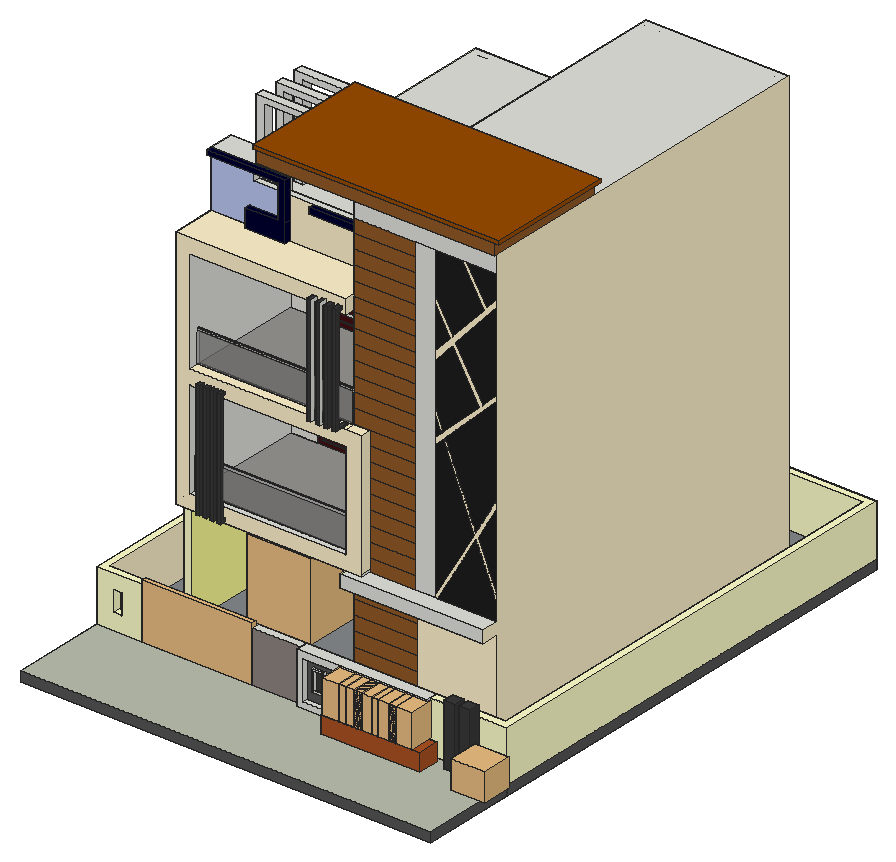
# SketchUp Ruby script. Lengths in inches.
U = 1.inch
M = Sketchup.active_model
def pt(a) = Geom::Point3d.new(a.map { |v| v * U })
def face(e, loops, mat)
  f = e.add_face(loops[0].map { |a| pt(a) })
  loops[1..].each { |l| e.add_face(l.map { |a| pt(a) }).erase! }
  f.material = f.back_material = mat if mat
  f
end
# faces: each face lists its corners as indices into pts; further lists are holes
def faces(e, pts, list, mat = nil) = list.each { |f| face(e, (f[0].is_a?(Array) ? f : [f]).map { |l| l.map { |i| pts[i] } }, mat) }
# xy, xz, yz: faces in a plane at the given z, y or x. An outline is a flat list of corners, or four numbers for a rectangle; further outlines are holes
def ring(l) = l.size == 4 ? [[l[0], l[1]], [l[2], l[1]], [l[2], l[3]], [l[0], l[3]]] : l.each_slice(2).to_a
def flat(e, list, mat, &to3) = list.each { |f| face(e, (f[0].is_a?(Array) ? f : [f]).map { |l| ring(l).map { |u, v| to3.(u, v) } }, mat) }
def xy(e, z, list, mat = nil) = flat(e, list, mat) { |x, y| [x, y, z] }
def xz(e, y, list, mat = nil) = flat(e, list, mat) { |x, z| [x, y, z] }
def yz(e, x, list, mat = nil) = flat(e, list, mat) { |y, z| [x, y, z] }
def lines(e, pts, list) = list.each { |a, b| e.add_line(pt(pts[a]), pt(pts[b])) }
# prism: a flat outline (further loops are holes) pulled along v
def prism(e, loops, v, mat = nil)
  f = face(e, loops, mat); d = Geom::Vector3d.new(v.map { |x| x * U })
  f.pushpull(f.normal.samedirection?(d) ? d.length : -d.length)
end
def box(e, o, s, mat = nil) = prism(e, [[o, [o[0] + s[0], o[1], o[2]], [o[0] + s[0], o[1] + s[1], o[2]], [o[0], o[1] + s[1], o[2]]]], [0, 0, s[2]], mat)
def at(x, y, z, deg = 0) = Geom::Transformation.translation(pt([x, y, z])) * Geom::Transformation.rotation(ORIGIN, Z_AXIS, deg.degrees)
def axes(o, x, y, z) = Geom::Transformation.new([*x, 0, *y, 0, *z, 0, *pt(o).to_a, 1])
def part(name) = M.definitions.add(name)
# library, detail: a bought-in or finely detailed component or shape, given as its bounding box
def library(name, o, s) = part(name).tap { |d| box(d.entities, o, s) }
def detail(e, o, s) = box(e.add_group.entities, o, s)
def put(e, d, t, mat = nil) = e.add_instance(d, t).tap { |i| i.material = mat if mat }
def group(e, t, mat = nil) = e.add_group.tap { |g| g.transformation = t; g.material = mat if mat }.entities
root = M.entities
M.materials.add("[Aluminum]").color = [179, 179, 179]
M.materials.add("[Blacktop Old 01]").color = [132, 136, 139]
M.materials.add("[Color C07]").color = [153, 76, 0]
M.materials.add("[Color C08]").color = [80, 51, 0]
M.materials.add("[Color D01]").color = [255, 242, 204]
M.materials.add("[Color E01]").color = [255, 255, 204]
M.materials.add("[Color E02]").color = [255, 255, 153]
M.materials.add("[Color I08]").color = [0, 0, 48]
M.materials.add("[Color L16]").color = [69, 15, 19]
M.materials.add("[Color M02]").color = [186, 198, 240]
M.materials.add("[Color M06]").color = [86, 86, 86]
M.materials.add("[Color M07]").color = [58, 58, 58]
M.materials.add("[Color M08]").color = [30, 30, 30]
M.materials.add("[Granite Light Gray]").color = [149, 148, 144]
M.materials.add("[Groundcover Rock Crushed Multi]").color = [143, 133, 129]
M.materials.add("[Marble Carrara Gold Floor Tile]").color = [225, 223, 217]
M.materials.add("[Pavers Square Brick]").color = [170, 82, 34]
M.materials.add("[Pavers with Grass Brick]").color = [187, 192, 176]
M.materials.add("[Translucent Glass Gray]").color = [128, 128, 128]
M.materials["[Translucent Glass Gray]"].alpha = 0.5
M.materials.add("[Wood Floor Parquet]").color = [145, 89, 39]
c1 = library("Plante",[-44.1,-44.03,0.04],[106.77,95.72,88.04])
c2 = library("Plant",[12.07,-11.84,0],[27.54,27.97,38.79])
c3 = part("Group\#1")
xy(c3.entities,0,[[0,0,64.375,6]],"[Color C08]")
xy(c3.entities,3.73,[[3.73,0,30.8125,6],[33.12,0,60.65,6]],"[Color C08]")
xy(c3.entities,60.65,[[3.73,0,30.8125,6],[33.12,0,60.65,6]],"[Color C08]")
xy(c3.entities,64.375,[[0,0,64.375,6]],"[Color C08]")
xz(c3.entities,0,[[[0,0,64.375,64.375],[33.12,3.73,60.65,60.65],[3.73,3.73,30.8125,60.65]]],"[Color C08]")
xz(c3.entities,0,[[3.73,3.73,30.8125,60.65],[33.12,3.73,60.65,60.65]],"[Translucent Glass Gray]")
xz(c3.entities,6,[[[0,0,64.375,64.375],[33.12,3.73,60.65,60.65],[3.73,3.73,30.8125,60.65]]],"[Color C08]")
yz(c3.entities,0,[[0,0,6,64.375]],"[Color C08]")
yz(c3.entities,3.73,[[0,3.73,6,60.65]],"[Color C08]")
yz(c3.entities,30.8125,[[0,3.73,6,60.65]],"[Color C08]")
yz(c3.entities,33.12,[[0,3.73,6,60.65]],"[Color C08]")
yz(c3.entities,60.65,[[0,3.73,6,60.65]],"[Color C08]")
yz(c3.entities,64.375,[[0,0,6,64.375]],"[Color C08]")
c4 = part("Group\#2")
xy(c4.entities,0,[[0,0,48,9.0625]])
xy(c4.entities,4.37,[[4.37,3.0625,43.63,9.0625]])
xy(c4.entities,4.37,[[4.37,0,43.63,3.0625]],"[Color L16]")
xy(c4.entities,11.3,[[4.37,3.0625,43.63,9.0625]])
xy(c4.entities,14.15,[[4.37,3.0625,43.63,9.0625]])
xy(c4.entities,23.32,[[4.37,3.0625,43.63,9.0625]])
xy(c4.entities,26.17,[[4.37,3.0625,43.63,9.0625]])
xy(c4.entities,35.95,[[4.37,3.0625,43.63,9.0625]])
xy(c4.entities,38.79,[[4.37,3.0625,43.63,9.0625]])
xy(c4.entities,49.95,[[4.37,3.0625,43.63,9.0625]])
xy(c4.entities,52.79,[[4.37,3.0625,43.63,9.0625]])
xy(c4.entities,63.01,[[4.37,3.0625,43.63,9.0625]])
xy(c4.entities,65.86,[[4.37,3.0625,43.63,9.0625]])
xy(c4.entities,75.2,[[4.37,3.0625,43.63,9.0625]])
xy(c4.entities,78.04,[[4.37,3.0625,43.63,9.0625]])
xy(c4.entities,79.63,[[4.37,3.0625,43.63,9.0625]])
xy(c4.entities,79.63,[[4.37,0,43.63,3.0625]],"[Color L16]")
xy(c4.entities,84,[[0,0,48,9.0625]],"[Color L16]")
xz(c4.entities,0,[[[0,0,48,84],[4.37,4.37,43.63,79.63]]],"[Color L16]")
xz(c4.entities,3.0625,[[4.37,11.3,43.63,14.15],[4.37,23.32,43.63,26.17],[4.37,35.95,43.63,38.79],[4.37,49.95,43.63,52.79],[4.37,63.01,43.63,65.86],
  [4.37,75.2,43.63,78.04]])
xz(c4.entities,3.0625,[[4.37,4.37,43.63,11.3],[4.37,14.15,43.63,23.32],[4.37,26.17,43.63,35.95],[4.37,38.79,43.63,49.95],[4.37,52.79,43.63,63.01],
  [4.37,65.86,43.63,75.2],[4.37,78.04,43.63,79.63]],"[Color L16]")
xz(c4.entities,9.0625,[[4.37,11.3,43.63,14.15],[4.37,23.32,43.63,26.17],[4.37,35.95,43.63,38.79],[4.37,49.95,43.63,52.79],[4.37,63.01,43.63,65.86],
  [4.37,75.2,43.63,78.04]])
xz(c4.entities,9.0625,[[[0,0,48,84],[4.37,4.37,43.63,79.63]],[4.37,4.37,43.63,11.3],[4.37,14.15,43.63,23.32],[4.37,26.17,43.63,35.95],[4.37,38.79,43.63,49.95],
  [4.37,52.79,43.63,63.01],[4.37,65.86,43.63,75.2],[4.37,78.04,43.63,79.63]],"[Color L16]")
yz(c4.entities,0,[[0,0,9.0625,84]],"[Color L16]")
yz(c4.entities,4.37,[[3.0625,4.37,9.0625,11.3],[3.0625,11.3,9.0625,14.15],[3.0625,14.15,9.0625,23.32],[3.0625,23.32,9.0625,26.17],[3.0625,26.17,9.0625,35.95],
  [3.0625,35.95,9.0625,38.79],[3.0625,38.79,9.0625,49.95],[3.0625,49.95,9.0625,52.79],[3.0625,52.79,9.0625,63.01],[3.0625,63.01,9.0625,65.86],
  [3.0625,65.86,9.0625,75.2],[3.0625,75.2,9.0625,78.04],[3.0625,78.04,9.0625,79.63]])
yz(c4.entities,4.37,[[0,4.37,3.0625,79.63]],"[Color L16]")
yz(c4.entities,43.63,[[3.0625,4.37,9.0625,11.3],[3.0625,11.3,9.0625,14.15],[3.0625,14.15,9.0625,23.32],[3.0625,23.32,9.0625,26.17],[3.0625,26.17,9.0625,35.95],
  [3.0625,35.95,9.0625,38.79],[3.0625,38.79,9.0625,49.95],[3.0625,49.95,9.0625,52.79],[3.0625,52.79,9.0625,63.01],[3.0625,63.01,9.0625,65.86],
  [3.0625,65.86,9.0625,75.2],[3.0625,75.2,9.0625,78.04],[3.0625,78.04,9.0625,79.63]])
yz(c4.entities,43.63,[[0,4.37,3.0625,79.63]],"[Color L16]")
yz(c4.entities,48,[[0,0,9.0625,84]],"[Color L16]")
c5 = library("Group\#3",[0,0,0],[121.6875,6,71.8125])
c6 = library("Group\#10",[0,0,0],[90.75,356.1,108.9])
xy(root,0,[[0,0,480,651.1875]],"[Color M07]")
xy(root,12,[[287.99,79.75,403.18,105.5],[238.86,105.5,390.47,111.1875],[0,111.1875,0,651.1875,480,651.1875,480,111.1875,390.47,111.1875,390.47,120.1875,471,120.1875,471,642.1875,9,642.1875,9,120.1875,52.9,120.1875,52.9,111.1875],[52.9,111.1875,182.06,120.1875],[182.06,111.1875,238.86,120.1875],
  [238.86,111.1875,390.47,120.1875],[[57,167.875,57,594.1875,423,594.1875,423,167.875,256,167.875,256,585.1875,66,585.1875,66,167.875],[262,173.875,414,585.1875]],[262,173.875,414,585.1875],[66,417.84,256,429.3125],[66,429.3125,256,585.1875]])
xy(root,12,[[[9,120.1875,471,642.1875],[57,167.875,57,594.1875,423,594.1875,423,167.875,256,167.875,256,417.84,66,417.84,66,167.875]]],"[Blacktop Old 01]")
xy(root,12,[[416.66,98.3125,429.54,111.1875],[434.29,98.3125,447.16,111.1875]],"[Color M07]")
xy(root,12,[[0,0,480,0,480,111.1875,447.16,111.1875,447.16,98.3125,434.29,98.3125,434.29,111.1875,429.54,111.1875,429.54,98.3125,416.66,98.3125,416.66,111.1875,390.47,111.1875,390.47,105.5,403.18,105.5,403.18,79.75,287.99,79.75,287.99,105.5,238.86,105.5,238.86,111.1875,0,111.1875]],"[Pavers with Grass Brick]")
xy(root,19.4375,[[246.3,105.5,383.03,105.5,383.03,111.1875,366.59,111.1875,366.59,109.625,364.32,109.625,364.32,111.1875,361.4,111.1875,361.4,109.625,359.13,109.625,359.13,111.1875,356.47,111.1875,356.47,109.625,354.19,109.625,354.19,111.1875,246.3,111.1875]])
xy(root,31.21,[[19.83,111.1875,30.08,131.8125]],"[Color E01]")
xy(root,31.33,[[254.64,108.125,267.81,111.1875],[273.01,108.125,286.18,111.1875],[290.07,108.125,303.25,111.1875]])
xy(root,32,[[287.99,79.75,403.18,105.5]],"[Pavers Square Brick]")
xy(root,33.1,[[256.41,108.125,266.03,111.1875],[274.78,108.125,284.41,111.1875],[291.85,108.125,301.47,111.1875]])
xy(root,54.17,[[256.41,108.125,266.03,111.1875],[274.78,108.125,284.41,111.1875],[291.85,108.125,301.47,111.1875]])
xy(root,55.27,[[19.83,111.1875,30.08,131.8125]],"[Color E01]")
xy(root,55.94,[[254.64,108.125,267.81,111.1875],[273.01,108.125,286.18,111.1875],[290.07,108.125,303.25,111.1875]])
xy(root,64.5625,[[246.3,105.5,246.3,111.1875,354.19,111.1875,354.19,109.625,356.47,109.625,356.47,111.1875,359.13,111.1875,359.13,109.625,361.4,109.625,361.4,111.1875,364.32,111.1875,364.32,109.625,366.59,109.625,366.59,111.1875,383.03,111.1875,383.03,105.5]])
xy(root,72,[[238.86,105.5,390.47,120.1875],[182.06,111.1875,238.86,120.1875]])
xy(root,72,[[0,111.1875,52.9,111.1875,52.9,120.1875,9,120.1875,9,642.1875,471,642.1875,471,120.1875,390.47,120.1875,390.47,111.1875,480,111.1875,480,651.1875,0,651.1875]],"[Color E01]")
xy(root,84.125,[[416.66,98.3125,429.54,111.1875],[434.29,98.3125,447.16,111.1875]],"[Color M07]")
xy(root,123.9375,[[256,147.4375,423,167.875]])
xy(root,138,[[256,147.4375,423,147.4375,423,167.875,274.6875,167.875,274.6875,155.375,256,155.375],[66,417.84,256,429.3125],[66,429.3125,256,585.1875]])
xy(root,138,[[57,155.375,66,167.875],[66,155.375,256,417.84]],"[Color D01]")
xy(root,139,[[262,173.875,414,585.1875]])
xy(root,139.68,[[85.6,149.375,89.97,155.375],[93.66,149.375,98.03,155.375],[102.03,149.375,106.41,155.375],[110.66,149.375,115.03,155.375]],"[Color M07]")
xy(root,143.8,[[85.6,152.375,89.97,155.375],[93.66,152.375,98.03,155.375],[102.03,152.375,106.41,155.375],[110.66,152.375,115.03,155.375]])
xy(root,144,[[66,308.75,256,585.1875]])
xy(root,149,[[153.55,302.75,256,308.75]])
xy(root,154.3125,[[73.6875,155.375,256,162.5],[73.6875,162.5,256,164.5]])
xy(root,154.3125,[[73.6875,164.5,256,164.5,256,302.75,153.55,302.75,153.55,308.75,105.55,308.75,105.55,302.75,73.6875,302.75]],"[Granite Light Gray]")
xy(root,184.64,[[181.68,302.75,230.68,308.75]])
xy(root,190.3125,[[73.6875,162.5,256,164.5]])
xy(root,193.3125,[[73.6875,162.5,256,164.5]],"[Aluminum]")
xy(root,233,[[105.55,302.75,153.55,308.75]])
xy(root,236.14,[[181.68,302.75,230.68,308.75]])
xy(root,258,[[262,173.875,414,585.1875]])
xy(root,269,[[73.6875,155.375,256,302.75]],"[Wood Floor Parquet]")
xy(root,272.79,[[85.6,152.375,89.97,155.375],[93.66,152.375,98.03,155.375],[102.03,152.375,106.41,155.9375],[110.66,152.375,115.03,155.3125]])
xy(root,276.3125,[[85.6,149.375,89.97,155.375],[93.66,149.375,98.03,155.375],[102.03,149.375,106.41,155.9375],[110.66,149.375,115.03,155.3125]],"[Color M07]")
xy(root,286,[[218.03,155.375,222.73,162.98],[228.22,155.375,232.92,162.98],[238.03,155.375,242.73,162.98],[247.34,155.375,252.04,162.98],[73.6875,166.3125,256,168.3125],
  [256,167.875,257.43,168.3125],[153.55,302.75,256,308.75]])
xy(root,286,[[73.6875,155.375,218.03,155.375,218.03,162.98,222.73,162.98,222.73,155.375,228.22,155.375,228.22,162.98,232.92,162.98,232.92,155.375,238.03,155.375,238.03,162.98,242.73,162.98,242.73,155.375,247.34,155.375,247.34,162.98,252.04,162.98,252.04,155.375,256,155.375,256,166.3125,73.6875,166.3125],[256,155.375,274.6875,167.875]],"[Color D01]")
xy(root,286,[[218.03,146.125,222.73,155.375],[228.22,146.125,232.92,155.375],[238.03,146.125,242.73,155.375],[247.34,146.125,252.04,155.375]],"[Color M07]")
xy(root,286,[[73.6875,168.3125,256,168.3125,256,302.75,153.55,302.75,153.55,308.75,105.55,308.75,105.55,302.75,73.6875,302.75]],"[Granite Light Gray]")
xy(root,287.8125,[[218.03,149.91,222.73,162.98],[228.22,149.91,232.92,162.98],[238.03,149.91,242.73,162.98],[247.34,149.91,252.04,162.98]],"[Color M07]")
xy(root,320.49,[[180.1,302.75,229.1,308.75]])
xy(root,322,[[73.6875,166.3125,256,168.3125]])
xy(root,323.8125,[[73.6875,166.3125,256,168.3125]],"[Aluminum]")
xy(root,370,[[105.55,302.75,153.55,308.75]])
xy(root,371.99,[[180.1,302.75,229.1,308.75]])
xy(root,400,[[262,173.875,414,585.1875]])
xy(root,406,[[73.6875,155.375,256,302.75]],"[Wood Floor Parquet]")
xy(root,414.375,[[218.03,146.125,222.73,156.16],[228.22,146.125,232.92,155.72],[238.03,146.125,242.73,155.66],[247.34,146.125,252.04,155.375]],"[Color M07]")
xy(root,423,[[101.625,201.32,101.625,207.7,107.3125,207.7,107.3125,215.57,256,215.57,256,207.7,148.8125,207.7,148.8125,201.32],[57,207.7,107.3125,236.82],[[107.3125,215.57,256,215.57,256,594.1875,57,594.1875,57,236.82,107.3125,236.82],[82.16,241.03,92.66,251.52],[82.16,270.03,92.66,280.52],[82.16,297.65,92.66,308.15]],[82.16,241.03,92.66,251.52],[82.16,270.03,92.66,280.52],
  [82.16,297.65,92.66,308.15]])
xy(root,423,[[57,155.375,256,155.375,256,207.7,148.8125,207.7,148.8125,201.32,101.625,201.32,101.625,207.7,57,207.7]],"[Color D01]")
xy(root,444.375,[[101.625,201.32,140.02,207.7]],"[Color I08]")
xy(root,463.85,[[176.5,201.32,256,207.7]],"[Color I08]")
xy(root,471,[[107.3125,207.7,256,215.57]])
xy(root,471,[[176.5,201.32,256,207.7]],"[Color I08]")
xy(root,483.625,[[57,201.32,140.02,207.7]],"[Color I08]")
xy(root,486.375,[[57,207.7,107.3125,236.82]])
xy(root,489.25,[[57,207.7,107.3125,236.82]])
xy(root,489.25,[[57,201.32,148.8125,207.7]],"[Color I08]")
xy(root,516.5,[[262,173.875,414,585.1875]])
xy(root,522.5,[[256,164.1875,423,167.875],[256,167.875,256,284.32,262,284.32,262,173.875,414,173.875,414,284.32,423,284.32,423,167.875],[256,284.32,423,309.53],[256,309.53,423,594.1875]])
xy(root,522.5,[[143.5625,164.1875,256,284.32],[143.5625,284.32,256,309.53]],"[Wood Floor Parquet]")
xy(root,532,[[92.66,241.03,143.5625,251.52],[92.66,270.03,143.5625,280.52],[92.66,297.65,146.84,308.15]])
xy(root,538.8125,[[143.5625,164.1875,423,309.53],[82.16,241.03,143.5625,251.52],[82.16,270.03,143.5625,280.52]])
xy(root,538.8125,[[143.5625,160,143.5625,164.1875,423,164.1875,423,309.53,431.6875,309.53,431.6875,160]],"[Wood Floor Parquet]")
xy(root,539.3125,[[82.16,297.65,146.84,308.15]])
xy(root,542.9375,[[143.5625,160,431.6875,309.53]],"[Color C07]")
xz(root,0,[[0,0,480,12]],"[Color M06]")
xz(root,79.75,[[287.99,12,403.18,32]],"[Pavers Square Brick]")
xz(root,98.3125,[[416.66,12,429.54,84.125],[434.29,12,447.16,84.125]],"[Color M07]")
xz(root,105.5,[[238.86,12,287.99,12,287.99,19.4375,246.3,19.4375,246.3,64.5625,383.03,64.5625,383.03,32,390.47,32,390.47,72,238.86,72],[287.99,12,390.47,12,390.47,32,383.03,32,383.03,19.4375,287.99,19.4375],[390.47,12,403.18,32],[287.99,19.4375,383.03,32]])
xz(root,108.125,[[[254.64,31.33,267.81,55.94],[256.41,33.1,266.03,54.17]],[[273.01,31.33,286.18,55.94],[274.78,33.1,284.41,54.17]],[[290.07,31.33,303.25,55.94],[291.85,33.1,301.47,54.17]]])
xz(root,109.625,[[354.19,19.4375,356.47,64.5625],[359.13,19.4375,361.4,64.5625],[364.32,19.4375,366.59,64.5625]],"[Color E02]")
xz(root,111.1875,[[416.66,12,429.54,72],[434.29,12,447.16,72]])
xz(root,111.1875,[[[0,12,52.9,72],[19.83,31.21,30.08,55.27]],[390.47,12,416.66,72],[429.54,12,434.29,72],[447.16,12,480,72]],"[Color E01]")
xz(root,111.1875,[[[246.3,19.4375,354.19,64.5625],[254.64,31.33,267.81,55.94],[273.01,31.33,286.18,55.94],[290.07,31.33,303.25,55.94]],[356.47,19.4375,359.13,64.5625],[361.4,19.4375,364.32,64.5625],[366.59,19.4375,383.03,64.5625]],"[Color M06]")
xz(root,111.1875,[[256.41,33.1,266.03,54.17],[274.78,33.1,284.41,54.17],[291.85,33.1,301.47,54.17],[416.66,72,429.54,84.125],[434.29,72,447.16,84.125]],"[Color M07]")
xz(root,111.1875,[[182.06,12,238.86,72]],"[Groundcover Rock Crushed Multi]")
xz(root,120.1875,[[182.06,12,238.86,72],[238.86,12,390.47,72],[390.47,12,471,72]])
xz(root,120.1875,[[9,12,52.9,72]],"[Color E01]")
xz(root,131.8125,[[19.83,31.21,30.08,55.27]])
xz(root,146.125,[[218.03,286,222.73,414.375],[228.22,286,232.92,414.375],[238.03,286,242.73,414.375],[247.34,286,252.04,414.375]],"[Color M07]")
xz(root,147.4375,[[256,123.9375,423,138]])
xz(root,149.375,[[85.6,139.68,89.97,276.3125],[93.66,139.68,98.03,276.3125],[102.03,139.68,106.41,276.3125],[110.66,139.68,115.03,276.3125]],"[Color M07]")
xz(root,149.91,[[218.03,287.8125,218.03,410.23,222.73,410.14,222.73,287.8125],[228.22,287.8125,228.22,410.03,232.92,409.9375,232.92,287.8125],[238.03,287.8125,238.03,409.83,242.73,409.74,242.73,287.8125],[247.34,287.8125,247.34,409.65,252.04,409.55,252.04,287.8125]],"[Color M07]")
xz(root,152.375,[[85.6,143.8,89.97,272.79],[93.66,143.8,98.03,272.79],[102.03,143.8,106.41,272.79],[110.66,143.8,115.03,272.79]],"[Color M07]")
xz(root,155.3125,[[110.66,272.79,115.03,276.3125]])
xz(root,155.375,[[[57,138,274.6875,138,274.6875,286,73.6875,286,73.6875,406,256,406,256,423,57,423],[73.6875,154.3125,256,269],[252.04,409.55,247.34,409.65,247.34,414.375,252.04,414.375],[85.6,139.68,89.97,143.8],[93.66,139.68,98.03,143.8],[102.03,139.68,106.41,143.8],[110.66,139.68,115.03,143.8],[93.66,272.79,98.03,276.3125],[85.6,272.79,89.97,276.3125]]],"[Color D01]")
xz(root,155.66,[[242.73,409.74,238.03,409.83,238.03,414.375,242.73,414.375]])
xz(root,155.72,[[232.92,409.9375,228.22,410.03,228.22,414.375,232.92,414.375]])
xz(root,155.9375,[[102.03,272.79,106.41,276.3125]])
xz(root,156.16,[[222.73,410.14,218.03,410.23,218.03,414.375,222.73,414.375]])
xz(root,160,[[143.5625,538.8125,431.6875,542.9375]],"[Color C07]")
xz(root,162.5,[[73.6875,190.3125,256,193.3125]],"[Aluminum]")
xz(root,162.5,[[73.6875,154.3125,256,190.3125]],"[Translucent Glass Gray]")
xz(root,162.98,[[218.03,286,222.73,287.8125],[228.22,286,232.92,287.8125],[238.03,286,242.73,287.8125],[247.34,286,252.04,287.8125]])
xz(root,164.1875,[[143.5625,522.5,423,538.8125]],"[Wood Floor Parquet]")
xz(root,164.5,[[73.6875,190.3125,256,193.3125]],"[Aluminum]")
xz(root,164.5,[[73.6875,154.3125,256,190.3125]],"[Translucent Glass Gray]")
xz(root,166.3125,[[73.6875,322,256,323.8125]],"[Aluminum]")
xz(root,166.3125,[[73.6875,286,256,322]],"[Translucent Glass Gray]")
xz(root,167.875,[[256,123.9375,423,132],[328.12,138,350.22,502.21],[256,139.875,274.6875,144],[256,144,274.6875,153.07],[256,153.07,274.6875,169.76],
  [256,169.76,274.6875,186.44],[256,186.44,274.6875,203.13],[256,203.13,274.6875,219.82],[256,219.82,274.6875,236.51],[256,236.51,274.6875,253.19],
  [256,253.19,274.6875,264],[256,264,274.6875,269.88],[256,269.88,274.6875,286],[256,502.21,423,522.5]])
xz(root,167.875,[[329.95,12,423,123.9375],[350.22,138,353.76,138,398.65,215.0625,423,156.34,423,165.49,400.56,218.35,423,256.875,423,264,398.9,222.27,362.1,308.94,423,368.77,423,374.36,406.25,358.29,374.36,412.86,423,467.99,423,474.66,410.79,461.25,386.61,502.21,383.55,502.21,408.59,458.84,371.37,417.97,350.22,454.15,350.22,448.47,368.95,415.3,350.22,394.74,350.22,385.5,371.9,410.07,402.9375,355.1,360,313.89,350.22,336.9375,350.22,331.83,358.33,312.28,350.22,304.49,350.22,297.27,360.4,307.27,397.01,219.01]],"[Color D01]")
xz(root,167.875,[[57,12,66,138]],"[Color E01]")
xz(root,167.875,[[350.22,138,397.01,219.01,360.4,307.27,350.22,297.27],[353.76,138,423,138,423,156.34,398.65,215.0625],[423,165.49,423,256.875,400.56,218.35],[398.9,222.27,423,264,423,368.77,362.1,308.94],[350.22,304.49,358.33,312.28,350.22,331.83],
  [360,313.89,402.9375,355.1,371.9,410.07,350.22,385.5,350.22,336.9375],[406.25,358.29,423,374.36,423,467.99,374.36,412.86],[350.22,394.74,368.95,415.3,350.22,448.47],[371.37,417.97,408.59,458.84,383.55,502.21,350.22,502.21,350.22,454.15],[410.79,461.25,423,474.66,423,502.21,386.61,502.21]],"[Color M08]")
xz(root,167.875,[[256,12,329.95,19.57],[256,19.57,329.95,36.26],[256,36.26,329.95,52.94],[256,52.94,329.95,69.63],[256,69.63,329.95,86.32],
  [256,86.32,329.95,103.01],[256,103.01,329.95,119.69],[256,119.69,329.95,123.9375],[274.6875,138,328.12,153.07],[274.6875,153.07,328.12,169.76],
  [274.6875,169.76,328.12,186.44],[274.6875,186.44,328.12,203.13],[274.6875,203.13,328.12,219.82],[274.6875,219.82,328.12,236.51],[274.6875,236.51,328.12,253.19],
  [274.6875,253.19,328.12,269.88],[274.6875,269.88,328.12,269.88,328.12,286.57,256,286.57,256,286,274.6875,286],[256,286.57,328.12,303.26],[256,303.26,328.12,319.94],[256,319.94,328.12,336.63],
  [256,336.63,328.12,353.32],[256,353.32,328.12,370.01],[256,370.01,328.12,386.69],[256,386.69,328.12,403.38],[256,403.38,328.12,420.07],
  [256,420.07,328.12,436.76],[256,436.76,328.12,453.44],[256,453.44,328.12,470.13],[256,470.13,328.12,486.82],[256,486.82,328.12,502.21]],"[Wood Floor Parquet]")
xz(root,168.3125,[[73.6875,322,256,323.8125]],"[Aluminum]")
xz(root,168.3125,[[73.6875,286,256,322]],"[Translucent Glass Gray]")
xz(root,173.875,[[262,12,414,132],[262,132,414,139],[262,400,414,516.5],[262,516.5,414,522.5]])
xz(root,201.32,[[101.625,423,148.8125,423,148.8125,489.25,57,489.25,57,483.625,140.02,483.625,140.02,444.375,101.625,444.375],[176.5,463.85,256,471]],"[Color I08]")
xz(root,207.7,[[140.02,444.375,148.8125,471],[176.5,463.85,256,471],[57,483.625,107.3125,486.375],[57,486.375,107.3125,489.25]])
xz(root,207.7,[[148.8125,423,256,423,256,463.85,176.5,463.85,176.5,471,148.8125,471]],"[Color D01]")
xz(root,207.7,[[140.02,471,140.02,483.625,107.3125,483.625,107.3125,489.25,148.8125,489.25,148.8125,471]],"[Color I08]")
xz(root,207.7,[[57,423,101.625,423,101.625,444.375,140.02,444.375,140.02,471,107.3125,471,107.3125,483.625,57,483.625]],"[Color M02]")
xz(root,215.57,[[107.3125,423,256,471]],"[Color D01]")
xz(root,236.82,[[57,486.375,107.3125,489.25]])
xz(root,236.82,[[57,423,107.3125,486.375]],"[Color M02]")
xz(root,241.03,[[82.16,423,92.66,423,92.66,532,143.5625,532,143.5625,538.8125,82.16,538.8125]])
xz(root,251.52,[[82.16,423,82.16,538.8125,143.5625,538.8125,143.5625,532,92.66,532,92.66,423]])
xz(root,270.03,[[82.16,423,92.66,423,92.66,532,143.5625,532,143.5625,538.8125,82.16,538.8125]])
xz(root,280.52,[[82.16,423,82.16,538.8125,143.5625,538.8125,143.5625,532,92.66,532,92.66,423]])
xz(root,297.65,[[82.16,423,92.66,423,92.66,532,146.84,532,146.84,539.3125,82.16,539.3125]])
xz(root,302.75,[[66,149,105.55,154.3125],[153.55,149,256,154.3125]])
xz(root,302.75,[[[73.6875,154.3125,105.55,154.3125,105.55,233,153.55,233,153.55,154.3125,256,154.3125,256,269,73.6875,269],[181.68,184.64,230.68,236.14]],[[73.6875,286,105.55,286,105.55,370,153.55,370,153.55,286,256,286,256,406,73.6875,406],[180.1,320.49,229.1,371.99]]],"[Marble Carrara Gold Floor Tile]")
xz(root,308.15,[[82.16,423,82.16,539.3125,146.84,539.3125,146.84,532,92.66,532,92.66,423]])
xz(root,308.75,[[66,144,66,149,105.55,149,105.55,154.3125,153.55,154.3125,153.55,149,256,149,256,144],[[66,149,66,269,256,269,256,149,153.55,149,153.55,233,105.55,233,105.55,149],[181.68,184.64,230.68,236.14]],[66,269,256,286],[[66,286,66,406,256,406,256,286,153.55,286,153.55,370,105.55,370,105.55,286],[180.1,320.49,229.1,371.99]]])
xz(root,309.53,[[414,522.5,423,538.8125],[414,538.8125,431.6875,542.9375]])
xz(root,309.53,[[143.5625,538.8125,414,542.9375]],"[Color C07]")
xz(root,309.53,[[143.5625,522.5,414,538.8125]],"[Wood Floor Parquet]")
xz(root,417.84,[[66,12,256,138]],"[Color E02]")
xz(root,429.3125,[[66,12,256,138]])
xz(root,585.1875,[[66,12,256,132],[262,12,414,132],[66,132,256,138],[262,132,414,139],[66,138,256,144],
  [262,139,280.5,144],[280.5,139,288.75,144],[288.75,139,414,144],[66,144,256,149],[262,144,414,258],
  [262,258,271.58,264],[271.58,258,297.02,264],[297.02,258,414,264],[262,264,414,400],[262,400,292.08,406],
  [292.08,400,308.27,406],[308.27,400,414,406],[262,406,414,516.5]])
xz(root,594.1875,[[57,12,57,406,256,406,256,522.5,423,522.5,423,12],[57,406,256,423]],"[Color D01]")
xz(root,642.1875,[[9,12,471,72]],"[Color E01]")
xz(root,651.1875,[[0,12,480,72]],"[Color E01]")
xz(root,651.1875,[[0,0,480,12]],"[Color M06]")
yz(root,0,[[111.1875,12,651.1875,72]],"[Color E01]")
yz(root,0,[[0,0,651.1875,12]],"[Color M06]")
yz(root,9,[[120.1875,12,642.1875,72]],"[Color D01]")
yz(root,19.83,[[111.1875,31.21,131.8125,55.27]],"[Color E01]")
yz(root,30.08,[[111.1875,31.21,131.8125,55.27]],"[Color E01]")
yz(root,52.9,[[111.1875,12,120.1875,72]])
yz(root,57,[[207.7,486.375,236.82,489.25]])
yz(root,57,[[167.875,12,167.875,138,155.375,138,155.375,423,594.1875,423,594.1875,12]],"[Color E01]")
yz(root,57,[[201.32,483.625,207.7,489.25]],"[Color I08]")
yz(root,57,[[207.7,423,236.82,486.375]],"[Color M02]")
yz(root,66,[[417.84,12,429.3125,132],[429.3125,12,585.1875,132],[417.84,132,429.3125,138],[429.3125,132,585.1875,138],[308.75,144,585.1875,149],
  [308.75,149,585.1875,269],[308.75,269,585.1875,286],[308.75,286,585.1875,406]])
yz(root,66,[[167.875,12,417.84,138]],"[Color E02]")
yz(root,73.6875,[[155.375,154.3125,162.5,154.3125,162.5,193.3125,164.5,193.3125,164.5,154.3125,302.75,154.3125,302.75,269,155.375,269],[162.5,154.3125,164.5,190.3125],[162.5,190.3125,164.5,193.3125],[155.375,286,166.3125,286,166.3125,323.8125,168.3125,323.8125,168.3125,286,302.75,286,302.75,406,155.375,406],[166.3125,286,168.3125,322],
  [166.3125,322,168.3125,323.8125]])
yz(root,82.16,[[241.03,423,251.52,538.8125],[270.03,423,280.52,538.8125],[297.65,423,308.15,539.3125]])
yz(root,85.6,[[149.375,139.68,149.375,276.3125,155.375,276.3125,155.375,272.79,152.375,272.79,152.375,143.8,155.375,143.8,155.375,139.68]],"[Color M07]")
yz(root,89.97,[[149.375,139.68,155.375,139.68,155.375,143.8,152.375,143.8,152.375,272.79,155.375,272.79,155.375,276.3125,149.375,276.3125]],"[Color M07]")
yz(root,92.66,[[241.03,423,251.52,532],[270.03,423,280.52,532],[297.65,423,308.15,532]])
yz(root,93.66,[[149.375,139.68,149.375,276.3125,155.375,276.3125,155.375,272.79,152.375,272.79,152.375,143.8,155.375,143.8,155.375,139.68]],"[Color M07]")
yz(root,98.03,[[149.375,139.68,155.375,139.68,155.375,143.8,152.375,143.8,152.375,272.79,155.375,272.79,155.375,276.3125,149.375,276.3125]],"[Color M07]")
yz(root,101.625,[[201.32,423,207.7,444.375]],"[Color I08]")
yz(root,102.03,[[149.375,139.68,149.375,276.3125,155.9375,276.3125,155.9375,272.79,152.375,272.79,152.375,143.8,155.375,143.8,155.375,139.68]],"[Color M07]")
yz(root,105.55,[[302.75,149,308.75,154.3125],[302.75,154.3125,308.75,233],[302.75,286,308.75,370]])
yz(root,106.41,[[149.375,139.68,155.375,139.68,155.375,143.8,152.375,143.8,152.375,272.79,155.9375,272.79,155.9375,276.3125,149.375,276.3125]],"[Color M07]")
yz(root,107.3125,[[215.57,423,236.82,486.375],[207.7,471,215.57,486.375],[207.7,486.375,215.57,489.25],[215.57,486.375,236.82,489.25]])
yz(root,110.66,[[149.375,139.68,149.375,276.3125,155.3125,276.3125,155.3125,272.79,152.375,272.79,152.375,143.8,155.375,143.8,155.375,139.68]],"[Color M07]")
yz(root,115.03,[[149.375,139.68,155.375,139.68,155.375,143.8,152.375,143.8,152.375,272.79,155.3125,272.79,155.3125,276.3125,149.375,276.3125]],"[Color M07]")
yz(root,140.02,[[201.32,444.375,207.7,483.625]],"[Color I08]")
yz(root,143.5625,[[160,538.8125,309.53,542.9375]],"[Color C07]")
yz(root,143.5625,[[164.1875,522.5,164.1875,538.8125,241.03,538.8125,241.03,532,251.52,532,251.52,538.8125,270.03,538.8125,270.03,532,280.52,532,280.52,538.8125,309.53,538.8125,309.53,522.5]],"[Wood Floor Parquet]")
yz(root,146.84,[[297.65,532,308.15,539.3125]])
yz(root,148.8125,[[201.32,423,207.7,444.375],[201.32,444.375,207.7,489.25]],"[Color I08]")
yz(root,153.55,[[302.75,149,308.75,154.3125],[302.75,154.3125,308.75,233],[302.75,286,308.75,370]])
yz(root,176.5,[[201.32,463.85,207.7,471]],"[Color I08]")
yz(root,180.1,[[302.75,320.49,308.75,371.99]])
yz(root,181.68,[[302.75,184.64,308.75,236.14]])
yz(root,182.06,[[111.1875,12,120.1875,72]])
yz(root,218.03,[[146.125,286,146.125,414.375,156.16,414.375,156.16,410.23,149.91,410.23,149.91,287.8125,162.98,287.8125,162.98,286]],"[Color M07]")
yz(root,222.73,[[146.125,286,162.98,286,162.98,287.8125,149.91,287.8125,149.91,410.14,156.16,410.14,156.16,414.375,146.125,414.375]])
yz(root,228.22,[[146.125,286,146.125,414.375,155.72,414.375,155.72,410.03,149.91,410.03,149.91,287.8125,162.98,287.8125,162.98,286]],"[Color M07]")
yz(root,229.1,[[302.75,320.49,308.75,371.99]])
yz(root,230.68,[[302.75,184.64,308.75,236.14]])
yz(root,232.92,[[146.125,286,162.98,286,162.98,287.8125,149.91,287.8125,149.91,409.9375,155.72,409.9375,155.72,414.375,146.125,414.375]])
yz(root,238.03,[[146.125,286,146.125,414.375,155.66,414.375,155.66,409.83,149.91,409.83,149.91,287.8125,162.98,287.8125,162.98,286]],"[Color M07]")
yz(root,238.86,[[105.5,12,111.1875,72],[111.1875,12,120.1875,72]])
yz(root,242.73,[[146.125,286,162.98,286,162.98,287.8125,149.91,287.8125,149.91,409.74,155.66,409.74,155.66,414.375,146.125,414.375]],"[Color M07]")
yz(root,246.3,[[105.5,19.4375,111.1875,64.5625]])
yz(root,247.34,[[146.125,286,146.125,414.375,155.375,414.375,155.375,409.65,149.91,409.65,149.91,287.8125,162.98,287.8125,162.98,286]],"[Color M07]")
yz(root,252.04,[[146.125,286,162.98,286,162.98,287.8125,149.91,287.8125,149.91,409.55,155.375,409.55,155.375,414.375,146.125,414.375]],"[Color M07]")
yz(root,254.64,[[108.125,31.33,111.1875,55.94]])
yz(root,256,[[417.84,12,429.3125,132],[429.3125,12,585.1875,132],[417.84,132,429.3125,138],[429.3125,132,585.1875,138],[167.875,144,302.75,154.3125],
  [302.75,144,308.75,149],[308.75,144,585.1875,264],[302.75,149,308.75,264],[155.375,154.3125,155.375,269,167.875,269,167.875,154.3125,164.5,154.3125,164.5,193.3125,162.5,193.3125,162.5,154.3125],[162.5,154.3125,164.5,190.3125],
  [167.875,154.3125,302.75,264],[162.5,190.3125,164.5,193.3125],[167.875,264,302.75,269],[302.75,264,308.75,269],[585.1875,264,594.1875,269],
  [167.875,269,308.75,286],[166.3125,286,167.875,322],[167.875,286,168.3125,322],[168.3125,286,168.3125,323.8125,167.875,323.8125,167.875,406,302.75,406,302.75,286],[302.75,286,308.75,406],
  [166.3125,322,167.875,323.8125],[167.875,322,168.3125,323.8125],[167.875,406,302.75,423],[302.75,406,308.75,423],[308.75,406,585.1875,423],
  [585.1875,406,594.1875,423],[167.875,423,167.875,522.5,594.1875,522.5,594.1875,423,215.57,423,215.57,471,201.32,471,201.32,463.85,207.7,463.85,207.7,423],[207.7,423,215.57,471],[201.32,463.85,207.7,471]])
yz(root,256,[[155.375,406,167.875,423]],"[Color D01]")
yz(root,256,[[167.875,12,167.875,123.9375,147.4375,123.9375,147.4375,138,417.84,138,417.84,12]],"[Color E02]")
yz(root,256.41,[[108.125,33.1,111.1875,54.17]])
yz(root,262,[[173.875,12,585.1875,132],[173.875,132,585.1875,139],[173.875,139,585.1875,144],[173.875,144,585.1875,258],[173.875,258,585.1875,264],
  [173.875,264,585.1875,400],[173.875,400,585.1875,406],[173.875,406,585.1875,516.5]])
yz(root,266.03,[[108.125,33.1,111.1875,54.17]])
yz(root,267.81,[[108.125,31.33,111.1875,55.94]])
yz(root,273.01,[[108.125,31.33,111.1875,55.94]])
yz(root,274.6875,[[155.375,138,167.875,139.875]])
yz(root,274.6875,[[155.375,139.875,167.875,286]],"[Color D01]")
yz(root,274.78,[[108.125,33.1,111.1875,54.17]])
yz(root,284.41,[[108.125,33.1,111.1875,54.17]])
yz(root,286.18,[[108.125,31.33,111.1875,55.94]])
yz(root,287.99,[[79.75,12,105.5,32]],"[Pavers Square Brick]")
yz(root,290.07,[[108.125,31.33,111.1875,55.94]])
yz(root,291.85,[[108.125,33.1,111.1875,54.17]])
yz(root,301.47,[[108.125,33.1,111.1875,54.17]])
yz(root,303.25,[[108.125,31.33,111.1875,55.94]])
yz(root,354.19,[[109.625,19.4375,111.1875,64.5625]],"[Color E02]")
yz(root,356.47,[[109.625,19.4375,111.1875,64.5625]],"[Color E02]")
yz(root,359.13,[[109.625,19.4375,111.1875,64.5625]],"[Color E02]")
yz(root,361.4,[[109.625,19.4375,111.1875,64.5625]],"[Color E02]")
yz(root,364.32,[[109.625,19.4375,111.1875,64.5625]],"[Color E02]")
yz(root,366.59,[[109.625,19.4375,111.1875,64.5625]],"[Color E02]")
yz(root,383.03,[[105.5,19.4375,111.1875,64.5625]])
yz(root,390.47,[[105.5,12,111.1875,72],[111.1875,12,120.1875,72]])
yz(root,403.18,[[79.75,12,105.5,32]],"[Pavers Square Brick]")
yz(root,414,[[173.875,12,585.1875,132],[173.875,132,585.1875,139],[173.875,139,585.1875,258],[173.875,258,585.1875,264],[173.875,264,585.1875,400],
  [173.875,400,585.1875,406],[173.875,406,585.1875,516.5]])
yz(root,416.66,[[98.3125,12,111.1875,84.125]],"[Color M07]")
yz(root,423,[[167.875,12,594.1875,12,594.1875,522.5,167.875,522.5,167.875,138,147.4375,138,147.4375,123.9375,167.875,123.9375]],"[Color D01]")
yz(root,423,[[164.1875,522.5,309.53,538.8125]],"[Wood Floor Parquet]")
yz(root,429.54,[[98.3125,12,111.1875,84.125]],"[Color M07]")
yz(root,431.6875,[[160,538.8125,309.53,542.9375]],"[Color C07]")
yz(root,434.29,[[98.3125,12,111.1875,84.125]],"[Color M07]")
yz(root,447.16,[[98.3125,12,111.1875,84.125]],"[Color M07]")
yz(root,471,[[120.1875,12,642.1875,72]],"[Color E01]")
yz(root,480,[[111.1875,12,651.1875,72]],"[Color E01]")
yz(root,480,[[0,0,111.1875,12],[111.1875,0,651.1875,12]],"[Color M06]")
p = [[252.04,149.91,409.55],[247.34,149.91,409.65],[247.34,155.375,409.65],[252.04,155.375,409.55],[242.73,149.91,409.74],[238.03,149.91,409.83],
  [238.03,155.66,409.83],[242.73,155.66,409.74],[232.92,149.91,409.9375],[228.22,149.91,410.03],[228.22,155.72,410.03],[232.92,155.72,409.9375],
  [222.73,149.91,410.14],[218.03,149.91,410.23],[218.03,156.16,410.23],[222.73,156.16,410.14],[256,585.1875,132],[256,594.1875,132],
  [66,302.75,149],[66,155.375,149],[256,585.1875,149],[256,594.1875,149],[256,585.1875,406],[66,585.1875,406],
  [66,302.75,406],[66,302.75,423],[66,308.75,406],[66,308.75,423],[66,585.1875,423],[77.625,585.1875,423],
  [256,399.03,280.08],[256,382.28,280.08],[256,308.75,277.5],[66,585.1875,277.5],[256,585.1875,277.5],[195.92,585.1875,286],
  [179.85,585.1875,286],[66,585.1875,286],[278.8125,585.1875,522.5],[278.8125,585.1875,516.5],[414,585.1875,516.5],[414,585.1875,522.5],
  [262,585.1875,516.5],[262,585.1875,522.5],[414,284.32,522.5],[414,284.32,526.5],[414,173.875,522.5],[414,173.875,526.5],
  [262,284.32,522.5],[262,284.32,526.5],[262,173.875,522.5],[262,173.875,526.5],[256,167.875,139.875],[256,165.3125,139.875],
  [256,167.875,136.38],[328.12,167.875,136.38],[256,167.875,2.88],[328.12,167.875,2.88],[416.58,-638.39,285.76],[416.58,-638.39,278.86]]
faces(root,p,[[0,1,2,3],[4,5,6,7],[8,9,10,11],[12,13,14,15]])
lines(root,p,[[16,17],[18,19],[20,21],[22,23],[24,25],[26,27],[23,28],[29,28],[30,31],[32,31],[33,34],[35,36],
  [36,37],[38,39],[40,41],[42,43],[44,45],[46,47],[48,49],[50,51],[52,53],[54,55],[56,57],[58,59]])
put(root,c1,axes([464.56,85.1875,14.3125],[0.3717,0,0],[0,0.3717,0],[0,0,0.3717]))
put(root,c2,at(276.88,91.87,32))
put(root,c2,at(295.95,91.87,32))
put(root,c2,at(314.2,91.87,32))
put(root,c2,at(335.2,91.87,32))
put(root,c2,at(354.57,91.87,32))
put(root,c3,axes([181.68,302.75,184.64],[0.76117,0,0],[0,0.68,0],[0,0,0.8]))
put(root,c4,at(105.55,302.75,286))
put(root,c4,axes([105.55,302.75,154.3125],[1,0,0],[0,0.9021,0],[0,0,0.93676]))
put(root,c3,axes([180.1,302.75,320.49],[0.76117,0,0],[0,0.68,0],[0,0,0.8]))
put(root,c5,axes([52.9,111.1875,11.25],[1.06145,0,0],[0,1,0],[0,0,0.91]))
put(root,c6,axes([179.09,366.39,13.08],[-0.83,0,0],[0,-0.4648,0],[0,0,0.83]))
